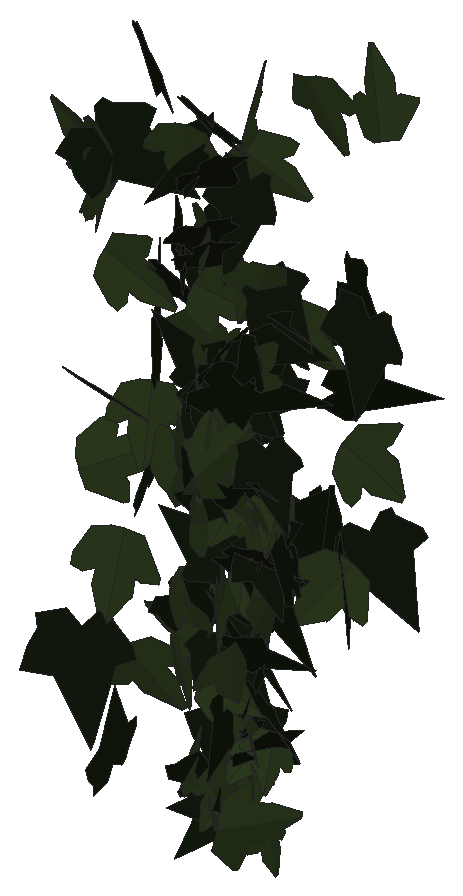
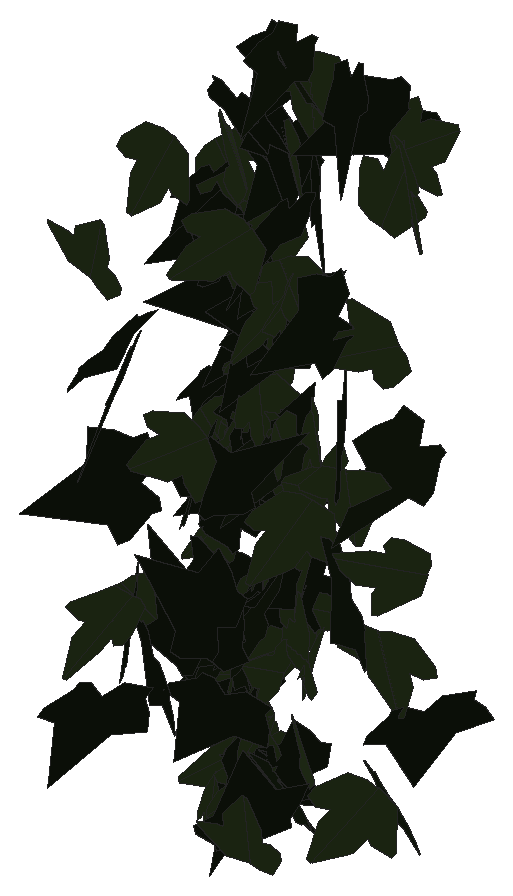
# SketchUp Ruby script. Lengths in inches.
U = 1.inch
M = Sketchup.active_model
def pt(a) = Geom::Point3d.new(a.map { |v| v * U })
def face(e, loops, mat)
  f = e.add_face(loops[0].map { |a| pt(a) })
  loops[1..].each { |l| e.add_face(l.map { |a| pt(a) }).erase! }
  f.material = f.back_material = mat if mat
  f
end
# faces: each face lists its corners as indices into pts; further lists are holes
def faces(e, pts, list, mat = nil) = list.each { |f| face(e, (f[0].is_a?(Array) ? f : [f]).map { |l| l.map { |i| pts[i] } }, mat) }
# xy, xz, yz: faces in a plane at the given z, y or x. An outline is a flat list of corners, or four numbers for a rectangle; further outlines are holes
def ring(l) = l.size == 4 ? [[l[0], l[1]], [l[2], l[1]], [l[2], l[3]], [l[0], l[3]]] : l.each_slice(2).to_a
def flat(e, list, mat, &to3) = list.each { |f| face(e, (f[0].is_a?(Array) ? f : [f]).map { |l| ring(l).map { |u, v| to3.(u, v) } }, mat) }
def xy(e, z, list, mat = nil) = flat(e, list, mat) { |x, y| [x, y, z] }
def xz(e, y, list, mat = nil) = flat(e, list, mat) { |x, z| [x, y, z] }
def yz(e, x, list, mat = nil) = flat(e, list, mat) { |y, z| [x, y, z] }
def lines(e, pts, list) = list.each { |a, b| e.add_line(pt(pts[a]), pt(pts[b])) }
# prism: a flat outline (further loops are holes) pulled along v
def prism(e, loops, v, mat = nil)
  f = face(e, loops, mat); d = Geom::Vector3d.new(v.map { |x| x * U })
  f.pushpull(f.normal.samedirection?(d) ? d.length : -d.length)
end
def box(e, o, s, mat = nil) = prism(e, [[o, [o[0] + s[0], o[1], o[2]], [o[0] + s[0], o[1] + s[1], o[2]], [o[0], o[1] + s[1], o[2]]]], [0, 0, s[2]], mat)
def at(x, y, z, deg = 0) = Geom::Transformation.translation(pt([x, y, z])) * Geom::Transformation.rotation(ORIGIN, Z_AXIS, deg.degrees)
def axes(o, x, y, z) = Geom::Transformation.new([*x, 0, *y, 0, *z, 0, *pt(o).to_a, 1])
def part(name) = M.definitions.add(name)
# library, detail: a bought-in or finely detailed component or shape, given as its bounding box
def library(name, o, s) = part(name).tap { |d| box(d.entities, o, s) }
def detail(e, o, s) = box(e.add_group.entities, o, s)
def put(e, d, t, mat = nil) = e.add_instance(d, t).tap { |i| i.material = mat if mat }
def group(e, t, mat = nil) = e.add_group.tap { |g| g.transformation = t; g.material = mat if mat }.entities
root = M.entities
M.materials.add("efeu1").color = [18, 25, 13]
M.materials.add("efeu2").color = [43, 57, 29]
c1 = part("ivyleaf_9")
p = [[1.54,2.16,1.25],[1.36,2.04,1.19],[-0.21,0.99,0.68],[-0.71,1.11,0.82],[-0.85,0.86,0.67],[-0.8,0.17,0.21],
  [-0.9,-0.01,0.1],[-0.67,-0.16,-0.02],[-0.08,-0.08,-0.05],[-0.03,-0.6,-0.4],[0.65,-0.88,-0.66],[0.83,-0.6,-0.49],
  [1.29,-0.42,-0.43],[1.8125,-0.07,-0.26],[1.21,0.44,0.15]]
faces(c1.entities,p,[[0,1,2,3,4,5,6,7,8,9,10,11,12,13,14]],"efeu1")
c2 = part("ivyleaf_10")
p = [[0,0.5,-0.03],[-0.0625,2.02,-0.43],[-0.19,2.01,-0.46],[-0.54,1.05,-0.29],[-0.52,0.625,-0.18],[-0.83,0.76,-0.28],
  [-1.16,0.64,-0.33],[-1.15,0.33,-0.24],[-0.77,-0.39,0.02],[-0.3,-0.51,0.16],[0.04,-0.48,0.23],[-0.02,2.01,-0.4375],
  [-0.06,2.01,-0.43],[0.04,-0.49,0.23],[0.67,-0.49,0.14],[1.38,0.36,-0.2],[1.375,0.51,-0.24],[0.81,0.65,-0.19],
  [0.62,0.59,-0.15],[0.6,1.09,-0.28],[0.5,1.23,-0.31]]
faces(c2.entities,p,[[0,1,2,3,4,5,6,7,8,9,10],[11,12,0,13,14,15,16,17,18,19,20]],"efeu2")
put(root,c1,axes([579.99,131,192.45],[-0.01957,0.48991,1.15271],[-0.1137,1.1474,-0.48958],[-1.24733,-0.11227,0.02654]))
put(root,c2,axes([580.24,128.31,204.4375],[-0.52364,0.1837,-0.84799],[-0.80775,0.25843,0.55478],[0.31681,0.96254,0.01288]))
put(root,c2,axes([578.97,129.95,193.13],[0.32519,0.0119,-0.99694],[0.86693,0.51451,0.28893],[0.49239,-0.91373,0.14971]))
put(root,c1,axes([579.42,128.66,188.26],[-0.26237,-1.03759,-0.42875],[0.09036,0.41936,-1.07016],[1.11904,-0.27713,-0.01411]))
put(root,c1,axes([579.42,129.07,196.2],[1.08328,0.17455,-0.23008],[-0.26758,0.27054,-1.05457],[-0.10867,1.07389,0.30307]))
put(root,c2,axes([579.81,129.8125,190.64],[1.13504,0.14642,-0.02052],[-0.02056,-0.00104,-1.14444],[-0.14641,1.13522,0.0016]))
put(root,c2,axes([579.66,130.89,186.53],[-0.83976,-0.23423,-0.58337],[0.55258,0.18912,-0.87136],[0.29974,-1.00486,-0.02801]))
put(root,c2,axes([580.11,129.37,203.25],[-0.27498,-0.6853,-0.78542],[-0.1463,-0.77887,0.73081],[-1.03205,0.29301,0.10566]))
put(root,c1,axes([580.47,130.78,196.45],[0.10656,-0.42793,1.17445],[0.01261,1.17902,0.42845],[-1.24992,-0.02458,0.10445]))
put(root,c2,axes([579.47,130.25,199.7],[0.40936,0.15052,0.95337],[0.88006,0.367,-0.43582],[-0.3963,0.97046,0.01695]))
put(root,c2,axes([580.57,128.2,203.96],[0.71952,-0.81204,-0.51588],[-0.31226,0.4122,-1.08436],[0.90996,0.78354,0.03581]))
put(root,c1,axes([580.64,130.2,207.02],[0.55512,0.03019,-0.85806],[-0.85627,0.09444,-0.55065],[0.06299,1.0176,0.07656]))
put(root,c2,axes([580.36,134.76,186.57],[1.00994,0.09858,0.09952],[-0.10551,0.05895,1.01242],[0.09213,-1.01312,0.06859]))
put(root,c1,axes([579.54,137.17,194.6],[0.29866,-0.2459,1.00252],[0.81255,-0.58764,-0.3862],[0.63661,0.8654,0.02262]))
put(root,c2,axes([580.43,130.46,195.48],[0.9275,0.41243,0.00353],[-0.00101,0.01098,-1.01501],[-0.41245,0.92744,0.01044]))
put(root,c1,axes([581.09,128.02,184.91],[-0.70967,0.37317,-0.49301],[-0.45816,0.18661,0.80076],[0.41522,0.84372,0.04095]))
put(root,c1,axes([580.57,128.09,205.32],[0.13199,-0.21575,-1.14344],[0.57244,1.01393,-0.12524],[1.01307,-0.54482,0.21974]))
put(root,c2,axes([581.51,131.1875,194.4],[-0.63576,-0.59603,-0.60846],[0.49127,0.36365,-0.86953],[0.6958,-0.80135,0.05798]))
put(root,c1,axes([581.19,130.16,199.92],[0.98851,-0.23007,0.12023],[0.11546,-0.0343,-1.0149],[0.2325,0.9952,-0.00718]))
put(root,c1,axes([581.46,134.37,190.53],[-0.31722,-0.48965,-0.84121],[0.52317,0.6603,-0.58164],[0.82078,-0.61013,0.04563]))
put(root,c2,axes([582.23,129.31,194.125],[0.13483,0.58742,-0.99],[0.1146,0.98497,0.60004],[1.14544,-0.16769,0.05649]))
put(root,c2,axes([583.18,128.64,195.375],[-0.37589,0.23738,0.81523],[-0.73679,0.35192,-0.44219],[-0.42201,-0.82586,0.04589]))
put(root,c2,axes([582.29,132.91,203.05],[-0.64027,-0.20766,-0.7731],[0.76009,0.15286,-0.67055],[0.25113,-0.9921,0.0585]))
put(root,c1,axes([583.27,128.41,202.66],[0.11869,0.02001,-0.96021],[-0.94363,0.18252,-0.11284],[0.17877,0.95015,0.04189]))
put(root,c1,axes([583.37,132.6,195.12],[-0.11956,-0.01736,1.01393],[-0.90582,-0.45718,-0.11464],[0.45592,-0.91288,0.03813]))
put(root,c2,axes([582.8,132.09,204.42],[0.62133,-0.80112,0.11044],[-0.06002,0.09321,1.01378],[-0.80646,-0.62415,0.00964]))
put(root,c1,axes([583.11,131.35,184.8125],[-0.6445,-0.56207,0.64956],[0.54362,0.36185,0.8525],[-0.66507,0.84045,0.06736]))
put(root,c2,axes([583.72,128.57,189.95],[-0.08194,0.10638,-0.86378],[-0.85823,0.13412,0.09794],[0.14444,0.85723,0.09187]))
put(root,c2,axes([583.09,128.48,189.06],[-0.38993,0.8103,-0.01689],[0.00416,-0.01675,-0.89923],[-0.81046,-0.38993,0.00352]))
put(root,c2,axes([583.22,128.56,205.79],[0.91701,0.265,-0.13186],[-0.23249,0.3792,-0.8548],[-0.18319,0.84528,0.4248]))
put(root,c1,axes([583.1,129.73,202.125],[0.39332,-0.57498,-0.76227],[-0.35472,0.67741,-0.694],[0.88647,0.52618,0.06051]))
put(root,c2,axes([582.63,129.52,189.21],[0.23321,-0.1254,1.09647],[1.03056,-0.37623,-0.26222],[0.39487,1.05598,0.03678]))
put(root,c1,axes([583.86,128.56,205.63],[-0.81448,0.46602,-0.0782],[0.06288,-0.04756,-0.93833],[-0.46834,-0.81685,0.01002]))
put(root,c2,axes([583.48,128.04,191.31],[-0.20321,0.66926,0.39902],[-0.15664,0.36885,-0.69845],[-0.76327,-0.25388,0.03711]))
put(root,c2,axes([582.91,133.96,197.27],[-0.61909,0.0106,-0.8286],[0.82369,-0.1054,-0.61677],[-0.09075,-1.02895,0.05464]))
put(root,c2,axes([583.74,128.82,199.6875],[0.76788,0.22349,-0.38903],[-0.44354,0.26203,-0.72495],[-0.06756,0.81996,0.3377]))
put(root,c1,axes([583.54,128.91,206.51],[0.78714,0.23407,-0.44365],[-0.49856,0.27414,-0.73993],[-0.05525,0.86097,0.35621]))
put(root,c1,axes([583.12,128.36,190.87],[0.06971,0.14102,-0.80543],[0.36579,0.71758,0.1573],[0.7313,-0.37237,-0.0019]))
put(root,c1,axes([584.13,128.64,198.21],[0.23099,-0.12422,0.84802],[-0.76924,0.35724,0.26186],[-0.37794,-0.80304,-0.01468]))
put(root,c2,axes([583.51,128.39,185.125],[0.5419,-0.55126,-0.04952],[0.04712,-0.0231,0.77282],[-0.55147,-0.54367,0.01737]))
put(root,c2,axes([583.79,129.01,194.98],[0.20428,-0.83413,0.15695],[0.04388,-0.15084,-0.85876],[0.84764,0.20883,0.00663]))
put(root,c1,axes([583.78,128.73,184.42],[-0.49509,0.67114,0.0543],[0.0293,-0.04586,0.83399],[0.6727,0.49595,0.00364]))
put(root,c2,axes([584.02,128.41,198.68],[0.06582,0.045,-0.9061],[-0.06842,0.90615,0.04003],[0.90464,0.06526,0.06895]))
put(root,c2,axes([584.2,128.55,194.23],[-0.8071,-0.09029,0.30162],[-0.29867,-0.04305,-0.81209],[0.09963,-0.86054,0.00898]))
put(root,c2,axes([584.09,136.54,203.18],[1.00505,-0.06574,0.43889],[-0.4335,0.08706,1.00576],[-0.09496,-1.09323,0.0537]))
put(root,c1,axes([583.48,134.6875,191.11],[-0.47844,-0.01674,-1.01868],[1.01701,-0.07482,-0.47643],[-0.06063,-1.12295,0.04693]))
put(root,c2,axes([584.27,128.18,203.18],[0.32812,-0.36418,-0.67779],[-0.40426,0.54535,-0.48872],[0.65467,0.51928,0.03792]))
put(root,c1,axes([583.82,128.97,194.57],[0.80304,0.24058,-0.26071],[-0.34055,0.34211,-0.73329],[-0.09936,0.77188,0.40626]))
put(root,c1,axes([584.68,128.43,192.56],[-0.13177,0.26432,0.80045],[-0.77523,0.2802,-0.22014],[-0.33107,-0.7613,0.1969]))
put(root,c1,axes([584.25,128.68,193.89],[0.59291,-0.15948,0.59776],[-0.55313,0.23422,0.61113],[-0.27713,-0.8087,0.05912]))
put(root,c1,axes([583.55,128.35,184.95],[0.31161,0.01773,0.71084],[0.69246,0.16881,-0.30776],[-0.16159,0.75756,0.05195]))
put(root,c1,axes([583.61,132.59,190.44],[-0.5325,0.01344,1.06052],[0.88952,-0.64061,0.45475],[0.57761,0.99893,0.27737]))
put(root,c1,axes([584.3125,127.97,203.49],[0.29203,0.71287,-0.20589],[-0.1656,-0.15306,-0.76486],[-0.7233,0.32287,0.09199]))
put(root,c2,axes([583.97,133.73,205.375],[-0.97129,0.14122,-0.33525],[0.32852,-0.07001,-0.98129],[-0.15624,-1.02514,0.02083]))
put(root,c2,axes([584.125,128.8,187.92],[0.09148,0.37178,-0.7102],[0.17117,0.68927,0.38287],[0.78314,-0.19408,-0.00073]))
put(root,c2,axes([584.14,128.7,198.53],[0.04351,0.39718,0.85176],[-0.10338,0.84952,-0.39085],[-0.9341,-0.07552,0.08293]))
put(root,c2,axes([584.05,135.47,192.67],[0.15293,0.80526,0.70289],[0.13945,0.68895,-0.81963],[-1.05974,0.20687,-0.00642]))
put(root,c1,axes([584.21,127.93,202.65],[0.52349,0.56688,0.19239],[0.06857,0.19711,-0.76737],[-0.5947,0.52173,0.08087]))
put(root,c2,axes([583.99,128.76,200.96],[0.26732,0.40819,0.80317],[0.28614,0.75593,-0.47942],[-0.8543,0.38092,0.09074]))
put(root,c1,axes([584.64,129.1875,185.38],[0.02501,-0.06347,-1.18131],[-0.85851,0.81196,-0.0618],[0.81393,0.85839,-0.02889]))
put(root,c2,axes([584.4,128.6,184.62],[-0.29787,0.72636,0.22086],[-0.08507,0.20383,-0.78507],[-0.75442,-0.30978,0.00132]))
put(root,c2,axes([584.47,127.79,193.98],[0.01783,0.38493,0.69312],[-0.21701,0.66919,-0.36605],[-0.76255,-0.18144,0.12038]))
put(root,c1,axes([584.82,128.73,184.62],[-0.84477,0.01906,-0.047],[0.047,-0.0004,-0.84498],[-0.01906,-0.84607,-0.00066]))
put(root,c1,axes([584.19,128.86,197.84],[-0.04415,-0.55109,-0.76334],[0.03674,0.76259,-0.55267],[0.94076,-0.05564,-0.01424]))
put(root,c1,axes([584.43,127.83,205.47],[0.44107,0.65403,0.17823],[0.06848,0.16856,-0.78802],[-0.67442,0.44486,0.03655]))
put(root,c2,axes([584.6875,128.72,186.09],[-0.08042,0.29698,0.77884],[-0.29144,0.72305,-0.3058],[-0.78093,-0.30042,0.03392]))
put(root,c1,axes([583.9,129.77,190.09],[0.89664,-0.74125,0.04984],[0.03985,-0.03001,-1.16336],[0.74185,0.89753,0.00226]))
put(root,c1,axes([584.23,128.79,194.9375],[0.55324,-0.65252,-0.33251],[-0.20166,0.26489,-0.85533],[0.70405,0.58862,0.0163]))
put(root,c2,axes([584.85,128.18,191.65],[0.12675,-0.44757,-0.80763],[-0.24971,0.76821,-0.46492],[0.88895,0.27961,-0.01545]))
put(root,c1,axes([584.63,128.65,198.16],[-0.08975,0.68526,-0.44885],[-0.28563,0.39702,0.66325],[0.76777,0.22781,0.19427]))
put(root,c2,axes([584.6875,128.61,185.29],[0.39752,0.5834,-0.34715],[-0.22225,-0.26828,-0.70535],[-0.64147,0.45448,0.02925]))
put(root,c1,axes([584.35,128.82,189.76],[0.05905,-0.51504,-0.68084],[0.07338,0.683,-0.51031],[0.85054,-0.02316,0.0913]))
put(root,c2,axes([584.93,128.47,185.39],[0.49278,-0.29878,-0.44575],[-0.33237,0.3052,-0.572],[0.4213,0.59024,0.07013]))
put(root,c1,axes([584.39,135.72,190.04],[-0.07789,-0.73338,-0.79222],[0.05205,0.7908,-0.73718],[1.0783,-0.09114,-0.02164]))
put(root,c1,axes([585.39,128.9,184.59],[-0.22669,-0.23004,-0.81395],[-0.57462,-0.57648,0.32296],[-0.62068,0.61771,-0.00172]))
put(root,c2,axes([584.85,128.58,195.68],[-0.22622,-0.81446,-0.02876],[0.00776,0.02769,-0.84529],[0.81493,-0.22636,0.00006]))
put(root,c2,axes([584.59,128.59,191.4],[-0.2118,0.67121,-0.47845],[0.10477,-0.46806,-0.70302],[-0.81759,-0.23385,0.03386]))
put(root,c1,axes([584.44,128.64,198.19],[0.05778,-0.36568,-0.82953],[0.02042,0.83153,-0.36514],[0.90633,0.00457,0.06111]))
put(root,c2,axes([584.72,128.64,187.1875],[-0.10657,0.81097,0.01659],[-0.00643,0.01588,-0.81793],[-0.81112,-0.10667,0.00431]))
put(root,c1,axes([584.97,127.84,199.42],[0.16422,0.65451,0.51705],[0.06742,0.51483,-0.67311],[-0.83137,0.17103,0.04754]))
put(root,c1,axes([584.84,134.13,199.07],[0.64059,-0.4603,-0.81916],[-0.66359,0.48029,-0.78881],[0.66524,0.92233,0.00195]))
put(root,c2,axes([585.23,128.26,184.89],[-0.58696,-0.00568,0.33988],[-0.33885,-0.04422,-0.58592],[0.02707,-0.67682,0.03543]))
put(root,c2,axes([584.82,128.56,197.17],[0.13163,0.84358,-0.05143],[-0.01338,-0.04997,-0.85377],[-0.84504,0.13219,0.00551]))
put(root,c2,axes([584.43,128.5,188.34],[0.2732,0.26336,0.74296],[0.54824,0.50149,-0.37936],[-0.56637,0.61247,-0.00884]))
put(root,c1,axes([584.64,128.88,187.46],[0.07898,-0.03445,-0.85971],[0.65679,-0.55527,0.08259],[-0.55579,-0.66107,-0.02457]))
put(root,c1,axes([585.39,128.96,188.22],[-0.10528,0.42318,0.78123],[-0.17586,0.76121,-0.43603],[-0.8709,-0.20487,-0.00639]))
put(root,c2,axes([585.05,128.49,194.71],[0.79597,0.09689,-0.23813],[-0.24031,0.00518,-0.80117],[-0.09133,0.83081,0.03276]))
put(root,c1,axes([584.97,129.36,204.58],[-0.86421,-0.16121,-0.56136],[0.54718,0.12708,-0.87887],[0.20422,-1.02266,-0.02073]))
put(root,c2,axes([584.96,127.47,196.21],[0.15293,0.26316,-1.09492],[0.35282,1.03814,0.29879],[1.06941,-0.38014,0.05801]))
put(root,c2,axes([585.2,128.1875,189.66],[-0.25071,-0.85925,-0.25407],[0.10111,0.23501,-0.89458],[0.8903,-0.26866,0.03005]))
put(root,c1,axes([584.6,134.03,195.57],[0.68195,0.32679,0.71701],[0.65349,0.29527,-0.75611],[-0.44027,0.94444,-0.0117]))
put(root,c1,axes([584.49,130.67,190.92],[-0.01501,-0.08732,-1.18105],[1.16215,0.22615,-0.03149],[0.22784,-1.15929,0.08282]))
put(root,c1,axes([585.88,128.73,193.25],[-0.43758,0.43099,0.4784],[-0.34055,0.336,-0.6142],[-0.54649,-0.55448,-0.00032]))
put(root,c1,axes([584.67,129.77,192.52],[-0.05594,0.05472,1.03283],[0.73201,-0.72862,0.07825],[0.73067,0.73415,0.00067]))
put(root,c2,axes([585.24,128.32,185.76],[-0.61243,-0.20672,-0.22388],[0.23223,0.00876,-0.64337],[0.19729,-0.65201,0.06234]))
put(root,c1,axes([585.39,128.01,195.32],[0.57159,0.53071,-0.277],[-0.22658,-0.16272,-0.77928],[-0.55411,0.61398,0.03291]))
put(root,c2,axes([586.04,128.3,194.22],[0.12983,-0.02553,-0.83585],[-0.75888,0.35173,-0.12862],[0.35128,0.76928,0.03107]))
put(root,c2,axes([585.12,128.57,184.2],[-0.41075,-0.29947,-0.57503],[0.54199,0.21496,-0.49909],[0.35579,-0.67318,0.09644]))
put(root,c2,axes([585.53,128.51,186],[0.62238,-0.40304,-0.12067],[0.01165,0.2319,-0.71445],[0.42055,0.59003,0.19838]))
put(root,c2,axes([585.625,128.9375,186.45],[-0.75168,-0.03931,0.04448],[0.03744,-0.7524,-0.03228],[0.04607,-0.02997,0.75202]))
put(root,c1,axes([584.82,127.99,198.48],[0.2621,0.46644,-1.03767],[0.52291,0.89632,0.53497],[1.01039,-0.58487,-0.00769]))
put(root,c2,axes([585.82,128.77,193.83],[0.05992,0.24872,-0.77648],[-0.03948,0.77854,0.24634],[0.81438,0.01944,0.06907]))
put(root,c2,axes([585.875,128.3,194.87],[-0.64997,0.31889,0.14994],[-0.13834,0.05842,-0.72394],[-0.32409,-0.66448,0.00831]))
put(root,c1,axes([585.17,128.55,189.68],[0.62081,0.02015,0.50427],[0.49854,0.09966,-0.61775],[-0.07838,0.79357,0.06478]))
put(root,c2,axes([586.12,132.07,190.93],[0.82476,0.19861,-0.59841],[-0.58057,-0.1451,-0.84832],[-0.24594,1.00859,-0.00421]))
put(root,c1,axes([585.4,128.1,193.03],[0.72943,0.19741,0.29731],[0.25896,0.17272,-0.75003],[-0.24557,0.76853,0.09219]))
put(root,c2,axes([586.1,128.6,202.32],[-0.36123,-0.6942,0.30882],[-0.13791,-0.27636,-0.78255],[0.74718,-0.38663,0.00487]))
put(root,c2,axes([585.96,128.28,187.28],[-0.41364,0.54895,0.06442],[-0.07075,0.02721,-0.68618],[-0.54817,-0.41774,0.03996]))
put(root,c2,axes([585.7,128.42,199.01],[-0.60685,-0.33163,0.40303],[0.36722,0.16792,0.69111],[-0.37089,0.70887,0.02483]))
put(root,c2,axes([585.875,128.75,191.69],[-0.11177,-0.24419,-0.71618],[0.26687,0.6647,-0.26828],[0.70804,-0.28909,-0.01193]))
put(root,c1,axes([585.63,128.98,188.25],[0.59395,-0.48433,0.04586],[0.02528,-0.04156,-0.76622],[0.48584,0.59427,-0.0162]))
put(root,c1,axes([585.87,128.72,193.26],[0.13899,-0.68762,-0.33008],[-0.07556,0.32145,-0.70147],[0.75899,0.15793,-0.00939]))
put(root,c1,axes([586.05,128.29,186.9],[0.41715,0.66579,0.23678],[0.12183,0.20308,-0.78567],[-0.69606,0.43455,0.00439]))
put(root,c2,axes([585.99,129.03,183.94],[0.02726,-0.71573,0.0047],[0.2651,0.00573,-0.66537],[0.66484,0.02706,0.26512]))
put(root,c1,axes([585.56,133,190.8],[0.12255,-0.07194,-1.03317],[0.97237,-0.35018,0.13972],[-0.35655,-0.97971,0.02593]))
put(root,c2,axes([586.2,128.94,191.32],[0.1763,-0.75873,-0.03852],[-0.00212,0.03906,-0.77891],[0.7597,0.17619,0.00677]))
put(root,c1,axes([586.09,128.31,199.27],[-0.11849,-0.18888,0.82813],[0.47099,0.68122,0.22277],[-0.70686,0.48557,0.00961]))
put(root,c2,axes([585.83,127.59,184.64],[-0.13175,-0.18646,-1.10218],[0.58524,0.93406,-0.22797],[0.9524,-0.59975,-0.01239]))
put(root,c1,axes([585.92,128.99,196.25],[0.11066,-0.78957,-0.29599],[-0.04199,0.29299,-0.79728],[0.84217,0.11836,-0.00086]))
put(root,c1,axes([586.13,128.97,201.85],[0.16774,-0.58045,-0.56606],[-0.11026,0.55635,-0.60316],[0.80324,0.19758,0.03541]))
put(root,c2,axes([586.22,128.89,186.83],[-0.349,-0.51556,0.36251],[0.3376,-0.50284,-0.39012],[0.5322,-0.01911,0.48519]))
put(root,c1,axes([586.04,128.29,200.39],[0.07682,0.06702,-0.85829],[0.09337,0.85597,0.0752],[0.85582,-0.09941,0.06884]))
put(root,c1,axes([586.11,133.4,198.68],[-0.00523,-1.02268,0.22363],[-0.02409,-0.22346,-1.02245],[1.04657,-0.01026,-0.02242]))
put(root,c2,axes([586.29,129.05,194.74],[-0.21643,-0.60173,0.45853],[0.31251,-0.50544,-0.51579],[0.68896,0.04024,0.378]))
put(root,c1,axes([586.83,128.96,192.42],[0.01488,-0.70606,0.94235],[-0.05191,0.94111,0.70595],[-1.17637,-0.05046,-0.01923]))
